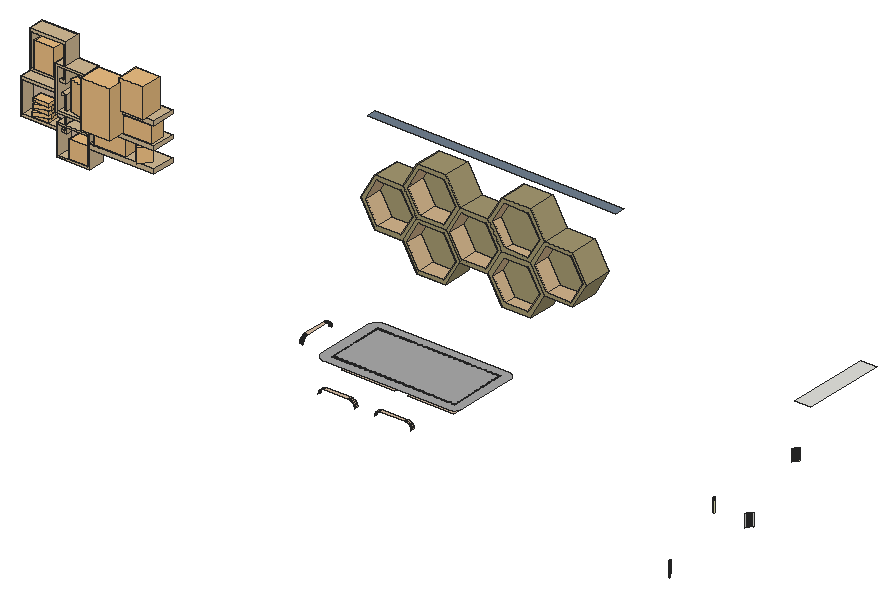
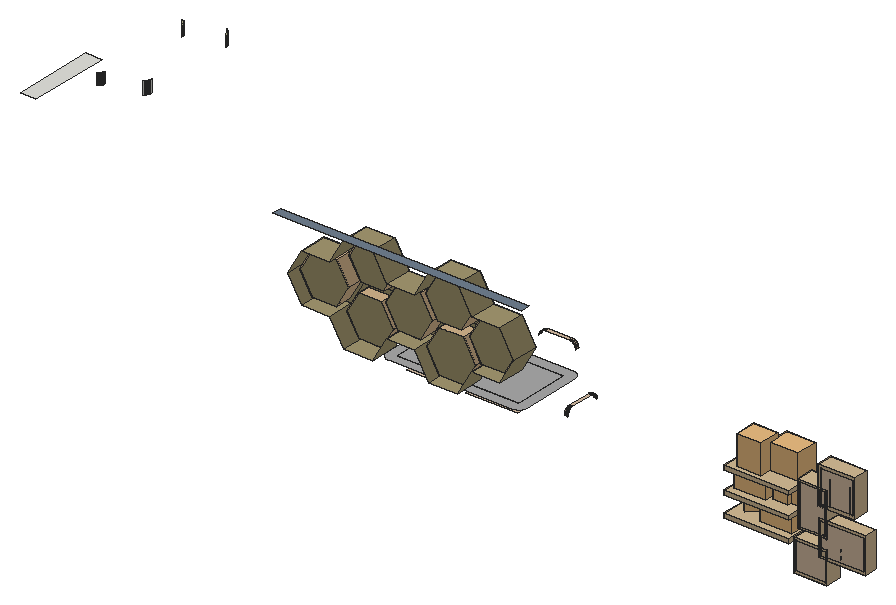
# SketchUp Ruby script. Lengths in inches.
U = 1.inch
M = Sketchup.active_model
def pt(a) = Geom::Point3d.new(a.map { |v| v * U })
def face(e, loops, mat)
  f = e.add_face(loops[0].map { |a| pt(a) })
  loops[1..].each { |l| e.add_face(l.map { |a| pt(a) }).erase! }
  f.material = f.back_material = mat if mat
  f
end
# faces: each face lists its corners as indices into pts; further lists are holes
def faces(e, pts, list, mat = nil) = list.each { |f| face(e, (f[0].is_a?(Array) ? f : [f]).map { |l| l.map { |i| pts[i] } }, mat) }
# xy, xz, yz: faces in a plane at the given z, y or x. An outline is a flat list of corners, or four numbers for a rectangle; further outlines are holes
def ring(l) = l.size == 4 ? [[l[0], l[1]], [l[2], l[1]], [l[2], l[3]], [l[0], l[3]]] : l.each_slice(2).to_a
def flat(e, list, mat, &to3) = list.each { |f| face(e, (f[0].is_a?(Array) ? f : [f]).map { |l| ring(l).map { |u, v| to3.(u, v) } }, mat) }
def xy(e, z, list, mat = nil) = flat(e, list, mat) { |x, y| [x, y, z] }
def xz(e, y, list, mat = nil) = flat(e, list, mat) { |x, z| [x, y, z] }
def yz(e, x, list, mat = nil) = flat(e, list, mat) { |y, z| [x, y, z] }
def lines(e, pts, list) = list.each { |a, b| e.add_line(pt(pts[a]), pt(pts[b])) }
# prism: a flat outline (further loops are holes) pulled along v
def prism(e, loops, v, mat = nil)
  f = face(e, loops, mat); d = Geom::Vector3d.new(v.map { |x| x * U })
  f.pushpull(f.normal.samedirection?(d) ? d.length : -d.length)
end
def box(e, o, s, mat = nil) = prism(e, [[o, [o[0] + s[0], o[1], o[2]], [o[0] + s[0], o[1] + s[1], o[2]], [o[0], o[1] + s[1], o[2]]]], [0, 0, s[2]], mat)
def at(x, y, z, deg = 0) = Geom::Transformation.translation(pt([x, y, z])) * Geom::Transformation.rotation(ORIGIN, Z_AXIS, deg.degrees)
def axes(o, x, y, z) = Geom::Transformation.new([*x, 0, *y, 0, *z, 0, *pt(o).to_a, 1])
def part(name) = M.definitions.add(name)
# library, detail: a bought-in or finely detailed component or shape, given as its bounding box
def library(name, o, s) = part(name).tap { |d| box(d.entities, o, s) }
def detail(e, o, s) = box(e.add_group.entities, o, s)
def put(e, d, t, mat = nil) = e.add_instance(d, t).tap { |i| i.material = mat if mat }
def group(e, t, mat = nil) = e.add_group.tap { |g| g.transformation = t; g.material = mat if mat }.entities
root = M.entities
M.materials.add("[0035_Tan]").color = [210, 180, 140]
M.materials.add("[0111_SlateGray]").color = [112, 128, 144]
M.materials.add("[0132_LightGray]").color = [169, 169, 169]
M.materials.add("[0136_Charcoal]").color = [35, 35, 35]
M.materials.add("[Color E01]").color = [255, 255, 204]
M.materials.add("[Formica Beige]").color = [211, 187, 149]
M.materials.add("[Formica Laminate Light]").color = [213, 189, 164]
M.materials.add("[Wood Lumber ButtJoined]").color = [164, 152, 112]
c1 = library("Books 284 012",[-3.9,-5.03,0],[7.8,10.06,1.71])
c2 = library("Books 008",[-5.8,-4.48,-0.01],[11.6,8.99,11.13])
c3 = library("Decoration 111 063",[-2.51,-1.28,-0.03],[5.02,2.53,10.66])
c4 = library("Books 297 001 004",[-3.55,-2.96,-0.03],[7.44,5.56,6.72])
c5 = library("Peperomia 450 001",[-6.6875,-10.1875,-9.42],[16.7,12.74,19.03])
c6 = library("Decorative Figures 02 65-28",[-3.68,-1.82,0],[7.71,3.84,6.72])
c7 = library("Books 120 040",[-9.2,-4.08,-0.03],[18.37,8.13,11.52])
c8 = library("Vase 20-16",[-4.28,-4.99,-0.02],[8.81,9.55,11.09])
c9 = library("Decorative Deer 209 004",[-1.58,-4.16,0],[3.36,7.25,10.63])
box(root,[60.47,188.06,62.6875],[37.56,13.62,2.5625],"[Formica Beige]")
box(root,[60.47,188.06,87.6875],[37.56,13.62,2.375],"[Formica Beige]")
box(root,[60.47,188.06,74.8125],[37.56,13.62,2.375],"[Formica Beige]")
xy(root,41.67,[[292.34,128.96,318.9375,155.08]],"[Formica Laminate Light]")
xy(root,41.75,[[254.38,128.96,284.55,155.08]],"[Formica Laminate Light]")
xy(root,48.6875,[[38.1,192.43,57.41,201.68]],"[Formica Beige]")
xy(root,49.31,[[[251.07,119.96,322.35,119.96,323.03,120.03,323.69,120.2,324.33,120.44,324.93,120.76,325.48,121.16,325.98,121.62,326.42,122.14,326.78,122.72,327.08,123.33,327.29,123.98,327.42,124.65,327.46,125.33,327.46,159.08,327.38,159.72,327.22,160.34,326.99,160.94,326.68,161.51,326.3,162.03,325.86,162.5,325.37,162.91,324.82,163.25,324.24,163.53,323.63,163.73,323,163.85,322.35,163.89,250.94,163.89,250.29,163.85,249.65,163.73,249.03,163.53,248.44,163.26,247.89,162.91,247.39,162.51,246.93,162.04,246.54,161.52,246.22,160.95,245.97,160.35,245.8,159.73,245.7,159.08,245.7,125.33,245.74,124.625,245.88,123.9375,246.11,123.27,246.42,122.64,246.81,122.06,247.27,121.53,247.8,121.07,248.38,120.68,249.01,120.37,249.68,120.14,250.37,120],[250.94,125.33,322.35,159.08]],[251.71,126.09,321.59,158.32]],"[0132_LightGray]")
xy(root,49.31,[[[250.94,125.33,322.35,159.08],[251.71,126.09,321.59,158.32]]],"[0136_Charcoal]")
xy(root,49.7,[[39.12,192.43,56.4,201.68]],"[Formica Beige]")
xy(root,50.4375,[[268.95,97.95,282.66,99.82],[301.11,97.95,315.66,99.82],[229.44,133.11,231.32,146.82]],"[Formica Laminate Light]")
xy(root,61.68,[[15.9,193.95,38.1,201.68],[38.1,193.95,39.12,201.68],[39.12,193.95,43.03,201.68]],"[Formica Beige]")
xy(root,62.97,[[17.1875,193.95,38.1,201.68],[38.1,193.95,39.12,201.68],[39.12,193.95,41.73,201.68]],"[Formica Beige]")
xy(root,65.98,[[39.12,192.43,56.4,201.68]],"[Formica Beige]")
xy(root,67,[[38.1,192.43,57.41,192.43,57.41,201.68,43.03,201.68,43.03,193.95,41.73,193.95,41.73,201.68,38.1,201.68],[41.73,193.95,43.03,201.68]],"[Formica Beige]")
xy(root,69.64,[[256.11,181.0625,272.5,197],[305.26,181.0625,321.64,197]],"[Wood Lumber ButtJoined]")
xy(root,71.52,[[257.2,181.0625,271.41,191.25]],"[0035_Tan]")
xy(root,72.08,[[306.67,181.0625,320.24,188.3125]],"[0035_Tan]")
xy(root,72.53,[[38.11,191.25,38.11,201.68,41.73,201.68,41.73,193.95,43.03,193.95,43.03,201.68,55.47,201.68,55.47,191.25],[41.73,193.95,43.03,201.68]],"[Formica Beige]")
xy(root,73.69,[[39.55,191.25,54.03,201.68]],"[Formica Beige]")
xy(root,80.83,[[17.1875,193.95,38.11,201.68],[38.11,193.95,41.73,201.68]],"[Formica Beige]")
xy(root,82.12,[[15.9,193.95,38.11,201.68],[38.11,193.95,39.55,201.68],[39.55,193.95,43.03,201.68]],"[Formica Beige]")
xy(root,83.83,[[231.54,181.0625,247.92,197],[280.6875,181.0625,297.07,197],[329.84,181.0625,346.22,197]],"[Wood Lumber ButtJoined]")
xy(root,85.88,[[331.02,181.0625,345.04,190.9375]],"[0035_Tan]")
xy(root,86.03,[[281.96,181.0625,295.8,190.8125]],"[0035_Tan]")
xy(root,86.16,[[232.89,181.0625,246.58,191.6875]],"[0035_Tan]")
xy(root,95.59,[[306.67,181.0625,320.24,188.3125]],"[0035_Tan]")
xy(root,96.14,[[257.2,181.0625,271.41,191.25]],"[0035_Tan]")
xy(root,96.8,[[39.55,191.25,54.03,201.68]],"[Formica Beige]")
xy(root,97.97,[[38.11,191.25,55.47,201.68]],"[Formica Beige]")
xy(root,100.16,[[257.35,181.0625,271.26,192.5625]],"[0035_Tan]")
xy(root,100.53,[[306.71,181.0625,320.2,186.75]],"[0035_Tan]")
xy(root,109.88,[[232.89,181.0625,246.58,191.6875]],"[0035_Tan]")
xy(root,110.01,[[281.96,181.0625,295.8,190.8125]],"[0035_Tan]")
xy(root,110.16,[[331.02,181.0625,345.04,190.9375]],"[0035_Tan]")
xy(root,112.21,[[231.54,181.0625,247.92,197],[280.6875,181.0625,297.07,197],[329.84,181.0625,346.22,197]],"[Wood Lumber ButtJoined]")
xy(root,119.9375,[[518.64,126.5625,527.89,173.6875]])
xy(root,123.88,[[306.71,181.0625,320.2,186.75]],"[0035_Tan]")
xy(root,124.25,[[257.35,181.0625,271.26,192.5625]],"[0035_Tan]")
xy(root,126.39,[[256.11,181.0625,272.5,197],[305.26,181.0625,321.64,197]],"[Wood Lumber ButtJoined]")
xy(root,129.75,[[214.53,197,358.53,202.625]],"[0111_SlateGray]")
xz(root,181.0625,[[[256.11,69.64,272.5,69.64,280.6875,83.83,272.5,98.02,256.11,98.02,247.92,83.83],[257.2,71.52,250.09,83.83,257.2,96.14,271.41,96.14,278.52,83.83,271.41,71.52]],[[305.26,69.64,321.64,69.64,329.84,83.83,321.64,98.02,305.26,98.02,297.07,83.83],[306.67,72.08,299.88,83.83,306.67,95.59,320.24,95.59,327.03,83.83,320.24,72.08]],[[231.54,83.83,247.92,83.83,256.11,98.02,247.92,112.21,231.54,112.21,223.35,98.02],[232.89,86.16,226.04,98.02,232.89,109.88,246.58,109.88,253.43,98.02,246.58,86.16]],[[280.6875,83.83,297.07,83.83,305.26,98.02,297.07,112.21,280.6875,112.21,272.5,98.02],[281.96,86.03,275.04,98.02,281.96,110.01,295.8,110.01,302.72,98.02,295.8,86.03]],[[329.84,83.83,346.22,83.83,354.41,98.02,346.22,112.21,329.84,112.21,321.64,98.02],[331.02,85.88,324.01,98.02,331.02,110.16,345.04,110.16,352.04,98.02,345.04,85.88]],
  [[256.11,98.02,272.5,98.02,280.6875,112.21,272.5,126.39,256.11,126.39,247.92,112.21],[257.35,100.16,250.4,112.21,257.35,124.25,271.26,124.25,278.21,112.21,271.26,100.16]],[[305.26,98.02,321.64,98.02,329.84,112.21,321.64,126.39,305.26,126.39,297.07,112.21],[306.71,100.53,299.97,112.21,306.71,123.88,320.2,123.88,326.9375,112.21,320.2,100.53]]],"[Wood Lumber ButtJoined]")
xz(root,186.75,[[306.71,100.53,320.2,100.53,326.9375,112.21,320.2,123.88,306.71,123.88,299.97,112.21]],"[Wood Lumber ButtJoined]")
xz(root,188.3125,[[306.67,72.08,320.24,72.08,327.03,83.83,320.24,95.59,306.67,95.59,299.88,83.83]],"[Wood Lumber ButtJoined]")
xz(root,190.8125,[[281.96,86.03,295.8,86.03,302.72,98.02,295.8,110.01,281.96,110.01,275.04,98.02]],"[Wood Lumber ButtJoined]")
xz(root,190.9375,[[331.02,85.88,345.04,85.88,352.04,98.02,345.04,110.16,331.02,110.16,324.01,98.02]],"[Wood Lumber ButtJoined]")
xz(root,191.25,[[[38.11,72.53,55.47,97.97],[39.55,73.69,54.03,96.8]]],"[Formica Beige]")
xz(root,191.25,[[257.2,71.52,271.41,71.52,278.52,83.83,271.41,96.14,257.2,96.14,250.09,83.83]],"[Wood Lumber ButtJoined]")
xz(root,191.6875,[[232.89,86.16,246.58,86.16,253.43,98.02,246.58,109.88,232.89,109.88,226.04,98.02]],"[Wood Lumber ButtJoined]")
xz(root,192.43,[[[38.1,48.6875,57.41,67],[39.12,49.7,56.4,65.98]]],"[Formica Beige]")
xz(root,192.5625,[[257.35,100.16,271.26,100.16,278.21,112.21,271.26,124.25,257.35,124.25,250.4,112.21]],"[Wood Lumber ButtJoined]")
xz(root,193.95,[[15.9,61.68,38.1,61.68,38.1,62.97,17.1875,62.97,17.1875,80.83,38.11,80.83,38.11,82.12,15.9,82.12],[38.1,61.68,39.12,62.97],[39.12,61.68,43.03,61.68,43.03,65.98,41.73,65.98,41.73,62.97,39.12,62.97],[41.73,65.98,43.03,67],[41.73,67,43.03,72.53],
  [41.73,72.53,43.03,73.69],[41.73,73.69,43.03,73.69,43.03,82.12,38.11,82.12,38.11,80.83,41.73,80.83]],"[Formica Beige]")
xz(root,201.68,[[[38.1,48.6875,57.41,67],[39.12,49.7,56.4,65.98]],[15.9,61.68,15.9,82.12,38.11,82.12,38.11,80.83,17.1875,80.83,17.1875,62.97,38.1,62.97,38.1,61.68],[38.1,61.68,39.12,62.97],[39.12,61.68,43.03,61.68,43.03,65.98,41.73,65.98,41.73,62.97,39.12,62.97],[38.1,62.97,41.73,67],
  [39.12,62.97,41.73,65.98],[41.73,65.98,43.03,67],[41.73,67,43.03,72.53],[38.11,72.53,41.73,72.53,41.73,73.69,39.55,73.69,39.55,80.83,38.11,80.83],[41.73,72.53,41.73,80.83,38.11,80.83,38.11,82.12,43.03,82.12,43.03,72.53],
  [43.03,72.53,43.03,73.69,54.03,73.69,54.03,96.8,39.55,96.8,39.55,82.12,38.11,82.12,38.11,97.97,55.47,97.97,55.47,72.53],[41.73,72.53,43.03,73.69],[38.11,80.83,39.55,82.12]],"[Formica Beige]")
xz(root,201.68,[[39.12,49.7,56.4,49.7,56.4,65.98,43.03,65.98,43.03,61.68,39.12,61.68],[17.1875,62.97,38.1,62.97,38.1,67,41.73,67,41.73,72.53,38.11,72.53,38.11,80.83,17.1875,80.83],[43.03,73.69,54.03,73.69,54.03,96.8,39.55,96.8,39.55,82.12,43.03,82.12]],"[Formica Laminate Light]")
yz(root,15.9,[[193.95,61.68,201.68,82.12]],"[Formica Beige]")
yz(root,17.1875,[[193.95,62.97,201.68,80.83]],"[Formica Beige]")
yz(root,38.1,[[192.43,48.6875,192.43,67,201.68,67,201.68,62.97,193.95,62.97,193.95,61.68,201.68,61.68,201.68,48.6875],[193.95,61.68,201.68,62.97]],"[Formica Beige]")
yz(root,38.11,[[191.25,72.53,191.25,97.97,201.68,97.97,201.68,89.77,192.62,89.77,192.62,88.3,201.68,88.3,201.68,82.12,193.95,82.12,193.95,80.83,201.68,80.83,201.68,72.53],[193.95,80.83,201.68,82.12],[192.62,88.3,201.68,89.77]],"[Formica Beige]")
yz(root,39.12,[[192.43,49.7,201.68,49.7,201.68,61.68,193.95,61.68,193.95,62.97,201.68,62.97,201.68,65.98,192.43,65.98],[193.95,61.68,201.68,62.97]],"[Formica Beige]")
yz(root,39.55,[[191.25,73.69,201.68,96.8]],"[Formica Beige]")
yz(root,41.73,[[193.95,62.97,201.68,65.98],[193.95,65.98,201.68,67],[193.95,67,201.68,72.53],[193.95,72.53,201.68,80.83]],"[Formica Beige]")
yz(root,43.03,[[193.95,61.68,201.68,67],[193.95,67,201.68,72.53],[193.95,72.53,201.68,73.69],[193.95,73.69,201.68,82.12]],"[Formica Beige]")
yz(root,54.03,[[191.25,73.69,201.68,96.8]],"[Formica Beige]")
yz(root,55.47,[[191.25,72.53,201.68,97.97]],"[Formica Beige]")
yz(root,56.4,[[192.43,49.7,201.68,65.98]],"[Formica Beige]")
yz(root,57.41,[[192.43,48.6875,201.68,67]],"[Formica Beige]")
p = [[265.3,99.82,47.23],[265.27,99.82,46.75],[265.27,97.95,46.75],[265.3,97.95,47.23],[297.92,99.82,47.26],[297.89,99.82,46.82],
  [297.89,97.95,46.82],[297.92,97.95,47.26],[319.1,99.82,46.82],[319.09,99.82,47.28],[319.09,97.95,47.28],[319.1,97.95,46.82],
  [231.32,150.47,47.23],[231.32,150.5,46.75],[229.44,150.5,46.75],[229.44,150.47,47.23],[286.47,99.82,46.86],[286.41,99.82,47.34],
  [286.41,97.95,47.34],[286.47,97.95,46.86],[231.32,129.3,46.86],[231.32,129.36,47.34],[229.44,129.36,47.34],[229.44,129.3,46.86],
  [265.39,99.82,47.7],[265.39,97.95,47.7],[231.32,150.38,47.7],[229.44,150.38,47.7],[286.29,99.82,47.8],[286.29,97.95,47.8],
  [298,99.82,47.69],[298,97.95,47.69],[319.02,99.82,47.74],[319.02,97.95,47.74],[231.32,129.48,47.8],[229.44,129.48,47.8],
  [265.55,99.82,48.16],[265.55,97.95,48.16],[298.13,99.82,48.12],[298.13,97.95,48.12],[318.89,99.82,48.1875],[318.89,97.95,48.1875],
  [231.32,150.22,48.16],[229.44,150.22,48.16],[286.11,99.82,48.25],[286.11,97.95,48.25],[231.32,129.65,48.25],[229.44,129.65,48.25],
  [298.3125,99.82,48.52],[298.3125,97.95,48.52],[265.76,99.82,48.59],[265.76,97.95,48.59],[285.88,99.82,48.67],[285.88,97.95,48.67],
  [318.7,99.82,48.61],[318.7,97.95,48.61],[231.32,129.89,48.67],[229.44,129.89,48.67],[231.32,150.01,48.59],[229.44,150.01,48.59],
  [298.54,99.82,48.89],[298.54,97.95,48.89],[266.03,99.82,48.99],[266.03,97.95,48.99],[318.45,99.82,49.01],[318.45,97.95,49.01],
  [231.32,149.74,48.99],[229.44,149.74,48.99],[285.6,99.82,49.05],[285.6,97.95,49.05],[231.32,130.17,49.05],[229.44,130.17,49.05],
  [298.8125,99.82,49.24],[298.8125,97.95,49.24],[266.35,99.82,49.36],[266.35,97.95,49.36],[318.15,99.82,49.37],[318.15,97.95,49.37],
  [231.32,149.42,49.36],[229.44,149.42,49.36],[285.27,99.82,49.4],[285.27,97.95,49.4],[231.32,130.5,49.4],[229.44,130.5,49.4],
  [299.125,99.82,49.55],[299.125,97.95,49.55],[266.71,99.82,49.68],[266.71,97.95,49.68],[284.9,99.82,49.71],[284.9,97.95,49.71],
  [317.8125,99.82,49.68],[317.8125,97.95,49.68],[231.32,130.87,49.71],[229.44,130.87,49.71],[231.32,149.06,49.68],[229.44,149.06,49.68],
  [299.47,99.82,49.82],[299.47,97.95,49.82],[267.11,99.82,49.94],[267.11,97.95,49.94],[284.5,99.82,49.97],[284.5,97.95,49.97],
  [317.43,99.82,49.95],[317.43,97.95,49.95],[231.32,131.27,49.97],[229.44,131.27,49.97],[231.32,148.66,49.94],[229.44,148.66,49.94],
  [299.85,99.82,50.05],[299.85,97.95,50.05],[267.54,99.82,50.16],[267.54,97.95,50.16],[317.02,99.82,50.16],[317.02,97.95,50.16],
  [231.32,148.23,50.16],[229.44,148.23,50.16],[284.0625,99.82,50.17],[284.0625,97.95,50.17],[231.32,131.7,50.17],[229.44,131.7,50.17],
  [300.26,99.82,50.23],[300.26,97.95,50.23],[268,99.82,50.3125],[268,97.95,50.3125],[283.61,99.82,50.32],[283.61,97.95,50.32],
  [300.68,99.82,50.36],[300.68,97.95,50.36],[316.58,99.82,50.3125],[316.58,97.95,50.3125],[231.32,132.16,50.32],[229.44,132.16,50.32],
  [231.32,147.77,50.3125],[229.44,147.77,50.3125],[268.47,99.82,50.41],[268.47,97.95,50.41],[283.14,99.82,50.41],[283.14,97.95,50.41],
  [316.125,99.82,50.41],[316.125,97.95,50.41],[231.32,132.63,50.41],[229.44,132.63,50.41],[231.32,147.3,50.41],[229.44,147.3,50.41],
  [268.95,99.82,50.4375],[268.95,97.95,50.4375],[282.66,99.82,50.4375],[282.66,97.95,50.4375],[301.11,99.82,50.4375],[301.11,97.95,50.4375],
  [315.66,99.82,50.4375],[315.66,97.95,50.4375],[231.32,133.11,50.4375],[229.44,133.11,50.4375],[231.32,146.82,50.4375],[229.44,146.82,50.4375],
  [247.92,197,83.83],[256.11,197,69.64],[256.11,181.0625,69.64],[247.92,181.0625,83.83],[272.5,197,69.64],[280.6875,197,83.83],
  [280.6875,181.0625,83.83],[272.5,181.0625,69.64],[297.07,197,83.83],[305.26,197,69.64],[305.26,181.0625,69.64],[297.07,181.0625,83.83],
  [321.64,197,69.64],[329.84,197,83.83],[329.84,181.0625,83.83],[321.64,181.0625,69.64],[250.09,181.0625,83.83],[257.2,181.0625,71.52],
  [257.2,191.25,71.52],[250.09,191.25,83.83],[271.41,181.0625,71.52],[278.52,181.0625,83.83],[278.52,191.25,83.83],[271.41,191.25,71.52],
  [299.88,181.0625,83.83],[306.67,181.0625,72.08],[306.67,188.3125,72.08],[299.88,188.3125,83.83],[320.24,181.0625,72.08],[327.03,181.0625,83.83],
  [327.03,188.3125,83.83],[320.24,188.3125,72.08],[530.07,21.39,85.38],[529.64,21.65,85.38],[529.64,21.65,78.19],[530.07,21.39,78.19],
  [529.24,21.96,85.38],[529.24,21.96,78.19],[528.89,22.32,85.38],[528.89,22.32,78.19],[528.58,22.72,85.38],[528.58,22.72,78.19],
  [528.32,23.15,85.38],[528.32,23.15,78.19],[528.12,23.61,85.38],[528.12,23.61,78.19],[527.97,24.1,85.38],[527.97,24.1,78.19],
  [527.89,24.59,85.38],[527.89,24.59,78.19],[527.89,78.67,85.38],[527.96,79.18,85.38],[527.96,79.18,78.19],[527.89,78.67,78.19],
  [528.1,79.67,85.38],[528.1,79.67,78.19],[528.3,80.14,85.38],[528.3,80.14,78.19],[528.55,80.58,85.38],[528.55,80.58,78.19],
  [528.86,80.99,85.38],[528.86,80.99,78.19],[529.22,81.36,85.38],[529.22,81.36,78.19],[529.61,81.68,85.38],[529.61,81.68,78.19],
  [530.05,81.95,85.38],[530.05,81.95,78.19],[223.35,197,98.02],[231.54,197,83.83],[231.54,181.0625,83.83],[223.35,181.0625,98.02],
  [257.2,181.0625,96.14],[257.2,191.25,96.14],[271.41,181.0625,96.14],[271.41,191.25,96.14],[306.67,181.0625,95.59],[306.67,188.3125,95.59],
  [320.24,181.0625,95.59],[320.24,188.3125,95.59],[346.22,197,83.83],[354.41,197,98.02],[354.41,181.0625,98.02],[346.22,181.0625,83.83],
  [324.01,181.0625,98.02],[331.02,181.0625,85.88],[331.02,190.9375,85.88],[324.01,190.9375,98.02],[345.04,181.0625,85.88],[352.04,181.0625,98.02],
  [352.04,190.9375,98.02],[345.04,190.9375,85.88],[275.04,181.0625,98.02],[281.96,181.0625,86.03],[281.96,190.8125,86.03],[275.04,190.8125,98.02],
  [295.8,181.0625,86.03],[302.72,181.0625,98.02],[302.72,190.8125,98.02],[295.8,190.8125,86.03],[226.04,181.0625,98.02],[232.89,181.0625,86.16],
  [232.89,191.6875,86.16],[226.04,191.6875,98.02],[246.58,181.0625,86.16],[253.43,181.0625,98.02],[253.43,191.6875,98.02],[246.58,191.6875,86.16],
  [530.28,53.51,104.19],[529.9,53.64,104.19],[529.9,53.64,97.75],[530.28,53.51,97.75],[529.53,53.81,104.19],[529.53,53.81,97.75],
  [529.19,54.02,104.19],[529.19,54.02,97.75],[528.88,54.28,104.19],[528.88,54.28,97.75],[528.61,54.57,104.19],[528.61,54.57,97.75],
  [528.375,54.9,104.19],[528.375,54.9,97.75],[528.18,55.25,104.19],[528.18,55.25,97.75],[528.03,55.625,104.19],[528.03,55.625,97.75],
  [527.9375,56.01,104.19],[527.9375,56.01,97.75],[527.89,56.41,104.19],[527.89,56.41,97.75],[527.89,112.29,104.19],[527.97,112.69,104.19],
  [527.97,112.69,97.75],[527.89,112.29,97.75],[528.1,113.09,104.19],[528.1,113.09,97.75],[528.26,113.47,104.19],[528.26,113.47,97.75],
  [528.46,113.84,104.19],[528.46,113.84,97.75],[528.69,114.18,104.19],[528.69,114.18,97.75],[528.96,114.5,104.19],[528.96,114.5,97.75],
  [529.25,114.79,104.19],[529.25,114.79,97.75],[529.58,115.05,104.19],[529.58,115.05,97.75],[529.92,115.28,104.19],[529.92,115.28,97.75],
  [530.29,115.47,104.19],[530.29,115.47,97.75],[231.54,197,112.21],[231.54,181.0625,112.21],[232.89,181.0625,109.88],[232.89,191.6875,109.88],
  [246.58,181.0625,109.88],[246.58,191.6875,109.88],[281.96,181.0625,110.01],[281.96,190.8125,110.01],[295.8,181.0625,110.01],[295.8,190.8125,110.01],
  [331.02,181.0625,110.16],[331.02,190.9375,110.16],[345.04,181.0625,110.16],[345.04,190.9375,110.16],[346.22,197,112.21],[346.22,181.0625,112.21],
  [250.4,181.0625,112.21],[257.35,181.0625,100.16],[257.35,192.5625,100.16],[250.4,192.5625,112.21],[271.26,181.0625,100.16],[278.21,181.0625,112.21],
  [278.21,192.5625,112.21],[271.26,192.5625,100.16],[299.97,181.0625,112.21],[306.71,181.0625,100.53],[306.71,186.75,100.53],[299.97,186.75,112.21],
  [320.2,181.0625,100.53],[326.9375,181.0625,112.21],[326.9375,186.75,112.21],[320.2,186.75,100.53],[256.11,197,126.39],[247.92,197,112.21],
  [247.92,181.0625,112.21],[256.11,181.0625,126.39],[257.35,181.0625,124.25],[257.35,192.5625,124.25],[271.26,181.0625,124.25],[271.26,192.5625,124.25],
  [280.6875,197,112.21],[272.5,197,126.39],[272.5,181.0625,126.39],[280.6875,181.0625,112.21],[305.26,197,126.39],[297.07,197,112.21],
  [297.07,181.0625,112.21],[305.26,181.0625,126.39],[306.71,181.0625,123.88],[306.71,186.75,123.88],[320.2,181.0625,123.88],[320.2,186.75,123.88],
  [329.84,197,112.21],[321.64,197,126.39],[321.64,181.0625,126.39],[329.84,181.0625,112.21],[42.04,201.68,97.97],[42.04,192.62,97.97],
  [43.32,192.62,97.97],[42.04,192.62,96.8],[42.04,201.68,96.8],[38.1,193.95,61.68],[38.1,193.95,61.66],[39.55,193.95,82.12],
  [39.55,193.95,80.87],[39.55,201.68,89.78],[39.55,192.62,89.78],[43.03,193.95,65.98],[43.04,193.95,65.98]]
faces(root,p,[[0,1,2,3],[4,5,6,7],[8,9,10,11],[12,13,14,15],[16,17,18,19],[20,21,22,23],[24,0,3,25],[26,12,15,27],
  [17,28,29,18],[30,4,7,31],[9,32,33,10],[21,34,35,22],[36,24,25,37],[38,30,31,39],[32,40,41,33],[42,26,27,43],
  [28,44,45,29],[34,46,47,35],[48,38,39,49],[50,36,37,51],[44,52,53,45],[40,54,55,41],[46,56,57,47],[58,42,43,59],
  [60,48,49,61],[62,50,51,63],[54,64,65,55],[66,58,59,67],[52,68,69,53],[56,70,71,57],[72,60,61,73],[74,62,63,75],
  [64,76,77,65],[78,66,67,79],[68,80,81,69],[70,82,83,71],[84,72,73,85],[86,74,75,87],[80,88,89,81],[76,90,91,77],
  [82,92,93,83],[94,78,79,95],[96,84,85,97],[98,86,87,99],[88,100,101,89],[90,102,103,91],[92,104,105,93],[106,94,95,107],
  [108,96,97,109],[110,98,99,111],[102,112,113,103],[114,106,107,115],[100,116,117,101],[104,118,119,105],[120,108,109,121],[122,110,111,123],
  [116,124,125,117],[126,120,121,127],[112,128,129,113],[118,130,131,119],[132,114,115,133],[134,122,123,135],[124,136,137,125],[128,138,139,129],
  [130,140,141,131],[142,132,133,143],[144,134,135,145],[136,146,147,137],[148,126,127,149],[138,150,151,139],[140,152,153,141],[154,142,143,155]],"[Formica Laminate Light]")
faces(root,p,[[156,157,158,159],[160,161,162,163],[164,165,166,167],[168,169,170,171],[224,225,226,227],[236,237,238,239],[308,224,227,309],[237,322,323,238],
  [340,341,342,343],[348,349,350,351],[352,353,354,355],[360,361,362,363]],"[Wood Lumber ButtJoined]")
faces(root,p,[[172,173,174,175],[176,177,178,179],[180,181,182,183],[184,185,186,187],[228,172,175,229],[177,230,231,178],[232,180,183,233],[185,234,235,186],
  [240,241,242,243],[244,245,246,247],[248,249,250,251],[252,253,254,255],[256,257,258,259],[260,261,262,263],[310,256,259,311],[261,312,313,262],
  [314,248,251,315],[253,316,317,254],[318,240,243,319],[245,320,321,246],[324,325,326,327],[328,329,330,331],[332,333,334,335],[336,337,338,339],
  [344,324,327,345],[329,346,347,330],[356,332,335,357],[337,358,359,338]],"[0035_Tan]")
faces(root,p,[[188,189,190,191],[189,192,193,190],[192,194,195,193],[194,196,197,195],[196,198,199,197],[198,200,201,199],[200,202,203,201],[202,204,205,203],
  [264,265,266,267],[265,268,269,266],[268,270,271,269],[270,272,273,271],[272,274,275,273],[274,276,277,275],[276,278,279,277],[278,280,281,279],
  [280,282,283,281],[282,284,285,283],[286,287,288,289],[287,290,291,288],[290,292,293,291],[292,294,295,293],[294,296,297,295],[296,298,299,297],
  [298,300,301,299],[300,302,303,301],[302,304,305,303],[304,306,307,305]],"[Color E01]")
faces(root,p,[[206,207,208,209],[207,210,211,208],[210,212,213,211],[212,214,215,213],[214,216,217,215],[216,218,219,217],[218,220,221,219],[220,222,223,221]])
lines(root,p,[[364,365],[365,366],[367,368],[369,370],[371,372],[373,374],[375,376]])
put(root,c1,axes([26.98,196.98,64.84],[-0.25774,0.70432,0],[-0.87336,-0.3196,0],[0,0,1.1397]),"[Formica Laminate Light]")
put(root,c1,axes([27.2,197.59,62.97],[0,0.75,0],[-0.93,0,0],[0,0,1.1397]),"[Formica Laminate Light]")
put(root,c1,axes([27.2,197.59,66.99],[0,0.75,0],[-0.93,0,0],[0,0,1.1397]),"[Formica Laminate Light]")
put(root,c1,axes([27.2,197.59,71],[0,0.75,0],[-0.93,0,0],[0,0,1.1397]),"[Formica Laminate Light]")
put(root,c1,axes([27.25,197.07,68.98],[-0.25774,0.70432,0],[-0.82096,-0.30043,0],[0,0,1.1397]),"[Formica Laminate Light]")
put(root,c2,axes([30.84,196.96,89.79],[0.99,0,0],[0,0.99,0],[0,0,1.3266]),"[Formica Laminate Light]")
g1 = group(root,at(25.72,201.68,94.39),"[Formica Laminate Light]")
xy(g1,-6.08,[[-3.52,-9.0625,17.6,0]],"[Formica Beige]")
xy(g1,-4.6,[[-2.24,-9.0625,16.32,0]],"[Formica Beige]")
xy(g1,14.12,[[-2.24,-9.0625,16.32,0]],"[Formica Beige]")
xy(g1,15.6,[[-3.52,-9.0625,17.6,0]],"[Formica Beige]")
xz(g1,-9.0625,[[[-3.52,-6.08,17.6,15.6],[-2.24,-4.6,16.32,14.12]]],"[Formica Beige]")
xz(g1,0,[[-2.24,-4.6,16.32,14.12]])
xz(g1,0,[[[-3.52,-6.08,17.6,15.6],[-2.24,-4.6,16.32,14.12]]],"[Formica Beige]")
yz(g1,-3.52,[[-9.0625,-6.08,0,15.6]],"[Formica Beige]")
yz(g1,-2.24,[[-9.0625,-4.6,0,14.12]],"[Formica Beige]")
yz(g1,16.32,[[-9.0625,-4.6,0,14.12]],"[Formica Beige]")
yz(g1,17.6,[[-9.0625,-6.08,0,15.6]],"[Formica Beige]")
put(root,c3,axes([48.7,195.61,73.71],[1.52048,-0.38868,0],[0.38884,1.52109,0],[0,0,1.57]),"[Formica Laminate Light]")
put(root,c4,axes([50.82,196.96,49.74],[-1.57135,0,0],[0,-1.41,0],[0,0,1.50969]),"[Formica Laminate Light]")
put(root,c5,axes([69.58,189.41,90.65],[1,0,0],[0,1,0],[0,0,1.4299]),"[Formica Laminate Light]")
put(root,c6,axes([71.13,192.04,77.1875],[1.16,0,0],[0,1,0],[0,0,1.23]),"[Formica Laminate Light]")
put(root,c7,axes([71.68,193.07,65.22],[1,0,0],[0,1,0],[0,0,0.76]),"[Formica Laminate Light]")
put(root,c8,axes([85.96,192.8,90.07],[1.5904,0,0],[0,1.2992,0],[0,0,1.5232]),"[Formica Laminate Light]")
put(root,c7,axes([86.85,192.9375,77.18],[1,0,0],[0,1,0],[0,0,0.81715]),"[Formica Laminate Light]")
put(root,c9,axes([90.32,191.58,65.25],[0.75813,-0.6521,0],[0.6521,0.75813,0],[0,0,0.75]),"[Formica Laminate Light]")
